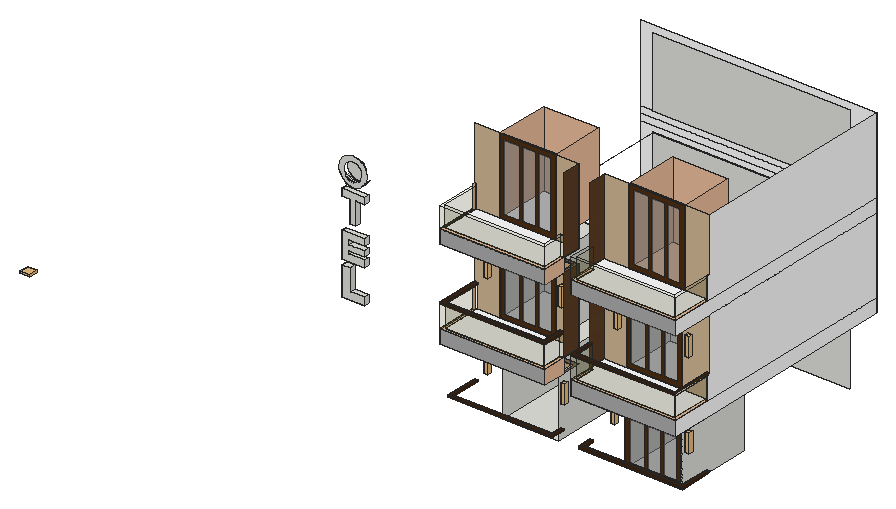
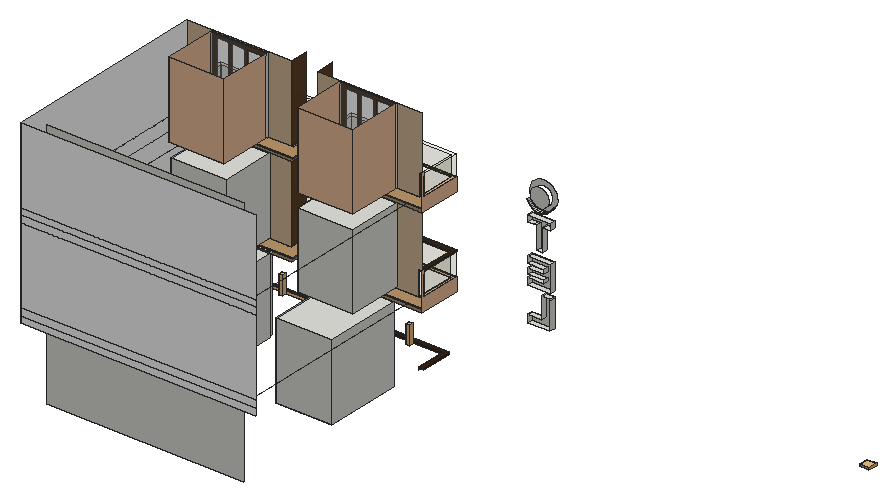
# SketchUp Ruby script. Lengths in inches.
U = 1.inch
M = Sketchup.active_model
def pt(a) = Geom::Point3d.new(a.map { |v| v * U })
def face(e, loops, mat)
  f = e.add_face(loops[0].map { |a| pt(a) })
  loops[1..].each { |l| e.add_face(l.map { |a| pt(a) }).erase! }
  f.material = f.back_material = mat if mat
  f
end
# faces: each face lists its corners as indices into pts; further lists are holes
def faces(e, pts, list, mat = nil) = list.each { |f| face(e, (f[0].is_a?(Array) ? f : [f]).map { |l| l.map { |i| pts[i] } }, mat) }
# xy, xz, yz: faces in a plane at the given z, y or x. An outline is a flat list of corners, or four numbers for a rectangle; further outlines are holes
def ring(l) = l.size == 4 ? [[l[0], l[1]], [l[2], l[1]], [l[2], l[3]], [l[0], l[3]]] : l.each_slice(2).to_a
def flat(e, list, mat, &to3) = list.each { |f| face(e, (f[0].is_a?(Array) ? f : [f]).map { |l| ring(l).map { |u, v| to3.(u, v) } }, mat) }
def xy(e, z, list, mat = nil) = flat(e, list, mat) { |x, y| [x, y, z] }
def xz(e, y, list, mat = nil) = flat(e, list, mat) { |x, z| [x, y, z] }
def yz(e, x, list, mat = nil) = flat(e, list, mat) { |y, z| [x, y, z] }
def lines(e, pts, list) = list.each { |a, b| e.add_line(pt(pts[a]), pt(pts[b])) }
# prism: a flat outline (further loops are holes) pulled along v
def prism(e, loops, v, mat = nil)
  f = face(e, loops, mat); d = Geom::Vector3d.new(v.map { |x| x * U })
  f.pushpull(f.normal.samedirection?(d) ? d.length : -d.length)
end
def box(e, o, s, mat = nil) = prism(e, [[o, [o[0] + s[0], o[1], o[2]], [o[0] + s[0], o[1] + s[1], o[2]], [o[0], o[1] + s[1], o[2]]]], [0, 0, s[2]], mat)
def at(x, y, z, deg = 0) = Geom::Transformation.translation(pt([x, y, z])) * Geom::Transformation.rotation(ORIGIN, Z_AXIS, deg.degrees)
def axes(o, x, y, z) = Geom::Transformation.new([*x, 0, *y, 0, *z, 0, *pt(o).to_a, 1])
def part(name) = M.definitions.add(name)
# library, detail: a bought-in or finely detailed component or shape, given as its bounding box
def library(name, o, s) = part(name).tap { |d| box(d.entities, o, s) }
def detail(e, o, s) = box(e.add_group.entities, o, s)
def put(e, d, t, mat = nil) = e.add_instance(d, t).tap { |i| i.material = mat if mat }
def group(e, t, mat = nil) = e.add_group.tap { |g| g.transformation = t; g.material = mat if mat }.entities
root = M.entities
M.materials.add("Generic").color = [68, 36, 11]
M.materials.add("Generic\#10").color = [214, 187, 153]
M.materials.add("Generic\#13").color = [239, 192, 158]
M.materials.add("Generic\#4").color = [186, 149, 106]
M.materials.add("Generic\#5").color = [175, 175, 175]
M.materials.add("Generic\#6").color = [117, 101, 81]
M.materials.add("[Color M00]").color = [255, 255, 255]
M.materials.add("[Translucent Glass Dark Green]").color = [86, 83, 28]
M.materials["[Translucent Glass Dark Green]"].alpha = 0.11
M.materials.add("[Translucent Glass Gray]1").color = [127, 127, 127]
M.materials["[Translucent Glass Gray]1"].alpha = 0.3
M.materials.add("[Wood Bamboo]").color = [81, 48, 19]
M.materials.add("[Wood Floor]").color = [91, 62, 36]
M.materials["[Wood Floor]"].alpha = 0.99
c1 = part("Group\#13")
xy(c1.entities,0,[[0,0,104.75,3]])
xy(c1.entities,142.8125,[[0,0,104.75,3]])
xz(c1.entities,0,[[8.08,8.08,37.11,134.73],[42.61,8.08,67.14,134.73],[72.39,8.08,96.67,134.73]],"[Translucent Glass Gray]1")
xz(c1.entities,0,[[[0,0,104.75,142.8125],[8.08,8.08,37.11,134.73],[42.61,8.08,67.14,134.73],[72.39,8.08,96.67,134.73]]],"[Wood Bamboo]")
xz(c1.entities,3,[[0,0,104.75,142.8125]],"[Translucent Glass Gray]1")
yz(c1.entities,0,[[0,0,3,142.8125]])
yz(c1.entities,104.75,[[0,0,3,142.8125]])
c2 = library("Tlon Light 450 Ceiling 152 006",[-8.86,-8.86,-3.78],[17.72,17.72,3.56])
c3 = library("Wall Lamp 298 005",[-4.37,-9,-20.45],[8.74,9.125,40.9])
xy(root,327.5625,[[458.2,140.75,562.95,286.875],[691.2,140.75,795.95,286.875]])
xy(root,372.75,[[404,78.3125,404,136.9375,409.82,136.9375,409.82,83.375,598,83.375,598,104.5,601.0625,104.5,601.0625,78.3125],[596.875,83.375,598,104.5]])
xy(root,372.75,[[650.9375,78.3125,650.9375,104.5,656.9375,104.5,656.9375,84.3125,842.4375,84.3125,842.4375,136.9375,848.4375,136.9375,848.4375,78.3125]],"Generic\#13")
xy(root,377.0625,[[404,78.3125,601.0625,78.3125,601.0625,104.5,596.875,104.5,596.875,83.375,409.82,83.375,409.82,140.75,404,140.75],[650.9375,78.3125,848.4375,78.3125,848.4375,136.9375,842.4375,136.9375,842.4375,84.3125,656.9375,84.3125,656.9375,104.5,650.9375,104.5],[842.4375,136.9375,848,140.75]],"Generic")
xy(root,470.375,[[458.2,140.75,562.95,286.875],[691.2,140.75,795.95,286.875]])
xy(root,470.375,[[[404,60.0625,601.0625,140.75],[409.34,65.4,595.73,131.6]],[[650.9375,60.0625,848,140.75],[655.73,64.86,843.21,132.14]]],"Generic\#6")
xy(root,471.6875,[[655.73,64.86,843.21,132.14],[409.34,65.4,595.73,131.6]],"Generic\#4")
xy(root,479.87,[[212.59,68.3125,254.57,78.3125]])
xy(root,494.05,[[228.04,68.3125,254.73,78.3125]])
xy(root,496.125,[[404,60.0625,404,136.9375,410,136.9375,410,66.0625,595.0625,66.0625,595.0625,104.5,601.0625,104.5,601.0625,60.0625],[650.9375,60.0625,650.9375,104.5,657.5625,104.5,657.5625,66.0625,842,66.0625,842,136.9375,848,136.9375,848,60.0625]],"Generic\#13")
xy(root,496.125,[[410,66.0625,595.0625,66.0625,595.0625,104.5,601.0625,104.5,601.0625,140.75,410,140.75],[657.5625,66.0625,842,66.0625,842,140.75,650.9375,140.75,650.9375,104.5,657.5625,104.5]],"[Color M00]")
xy(root,497.125,[[452.52,140.75,557.27,243.1875],[691.2,140.75,795.95,243.1875]])
xy(root,534.23,[[212.45,68.3125,227.88,78.3125]])
xy(root,538.125,[[404,60.0625,404,136.9375,410,136.9375,410,66.0625,595.0625,66.0625,595.0625,104.5,601.0625,104.5,601.0625,60.0625],[650.9375,60.0625,650.9375,104.5,657.5625,104.5,657.5625,66.0625,842,66.0625,842,136.9375,848,136.9375,848,60.0625]])
xy(root,541.4375,[[404,60.0625,601.0625,60.0625,601.0625,104.5,595.0625,104.5,595.0625,66.0625,410,66.0625,410,140.75,404,140.75],[650.9375,60.0625,848,60.0625,848,140.75,842,140.75,842,66.0625,657.5625,66.0625,657.5625,104.5,650.9375,104.5]],"Generic")
xy(root,543.68,[[212.13,68.3125,254.57,78.3125]])
xy(root,556.18,[[224.88,68.3125,254.57,78.3125]])
xy(root,561.8,[[224.88,68.3125,254.57,78.3125]])
xy(root,572.3,[[224.88,68.3125,254.57,78.3125]])
xy(root,579.92,[[224.88,68.3125,254.57,78.3125]])
xy(root,592.36,[[212.13,68.3125,254.57,78.3125]])
xy(root,608.06,[[226.26,68.3125,238.26,78.3125]])
xy(root,640.125,[[452.52,140.75,557.27,243.1875],[691.2,140.75,795.95,243.1875]])
xy(root,640.125,[[[404,60.0625,601.0625,140.75],[408.75,64.8125,596.3125,132.1875]],[[650.9375,60.0625,848,140.75],[655.28,64.4,843.66,132.6]]],"Generic\#6")
xy(root,641.4375,[[655.28,64.4,843.66,132.6],[408.75,64.8125,596.3125,132.1875]],"Generic\#4")
xy(root,650.42,[[210.88,68.3125,226.26,78.3125],[238.26,68.3125,242.57,78.3125],[242.57,68.3125,254.57,78.3125]])
xy(root,662.42,[[210.88,68.3125,254.57,78.3125]])
xy(root,665.875,[[404,60.0625,404,136.9375,408.8125,136.9375,408.8125,66.0625,596,66.0625,596,104.5,601.0625,104.5,601.0625,60.0625],[650.9375,60.0625,650.9375,104.5,657.6875,104.5,657.6875,66.0625,842,66.0625,842,136.9375,848,136.9375,848,60.0625],[696.14,140.75,800.89,243.1875]],"Generic\#13")
xy(root,665.875,[[408.8125,66.0625,596,66.0625,596,104.5,601.0625,104.5,601.0625,140.75,557.27,140.75,557.27,243.1875,452.52,243.1875,452.52,140.75,408.8125,140.75],[657.6875,66.0625,842,66.0625,842,140.75,650.9375,140.75,650.9375,104.5,657.6875,104.5]],"[Color M00]")
xz(root,60.0625,[[404,538.125,601.0625,541.4375],[650.9375,538.125,848,541.4375]],"Generic")
xz(root,60.0625,[[404,470.375,601.0625,496.125],[650.9375,470.375,848,496.125],[404,640.125,601.0625,665.875],[650.9375,640.125,848,665.875]],"Generic\#5")
xz(root,60.0625,[[404,496.125,601.0625,538.125],[650.9375,496.125,848,538.125],[404,665.875,601.0625,704.1875],[650.9375,665.875,848,704.1875]],"[Translucent Glass Dark Green]")
xz(root,64.4,[[655.28,640.125,843.66,641.4375]])
xz(root,64.8125,[[408.75,640.125,596.3125,641.4375]])
xz(root,64.86,[[655.73,470.375,843.21,471.6875]])
xz(root,65.4,[[409.34,470.375,595.73,471.6875]])
xz(root,66.0625,[[410,538.125,595.0625,541.4375],[657.5625,538.125,842,541.4375]],"Generic")
xz(root,66.0625,[[410,496.125,595.0625,538.125],[657.5625,496.125,842,538.125],[408.8125,665.875,596,704.1875],[657.6875,665.875,842,704.1875]],"[Translucent Glass Dark Green]")
xz(root,68.3125,[[212.59,479.87,254.57,479.87,254.73,494.05,228.04,494.05,227.88,534.23,212.45,534.23,212.59,531.7],[212.13,543.68,254.57,543.68,254.57,556.18,224.88,556.18,224.88,561.8,254.57,561.8,254.57,572.3,224.88,572.3,224.88,579.92,254.57,579.92,254.57,592.36,212.13,592.36],[226.26,608.06,238.26,608.06,238.26,650.42,254.57,650.42,254.57,662.42,210.88,662.42,210.88,650.42,226.26,650.42],[[233.53,671.96,236.44,672.22,239.27,672.93,242.09,673.69,244.76,674.89,247.27,676.38,249.6,678.15,251.72,680.16,253.6,682.4,255.21,684.83,256.55,687.44,257.58,690.17,258.3,693,258.7,695.9,258.78,698.82,258.52,701.73,257.95,704.59,257.05,707.375,255.85,710.04,254.36,712.55,252.59,714.88,250.58,717,248.34,718.88,245.91,720.5,243.3,721.83,240.57,722.87,237.74,723.59,234.84,723.99,231.92,724.0625,229.01,723.81,226.15,723.23,223.36,722.33,220.7,721.13,218.1875,719.64,215.86,717.88,213.74,715.86,211.86,713.625,210.24,711.19,208.91,708.59,207.875,705.86,207.15,703.02,206.75,700.13,206.68,697.21,206.93,694.3,207.51,691.43,208.4,688.65,209.61,685.98,211.1,683.47,212.86,681.14,214.875,679.02,217.11,677.14,219.55,675.53,222.15,674.19,224.88,673.16,227.72,672.4375,230.61,672.04],[233.26,680.77,231.33,680.82,229.41,681.08,227.53,681.56,225.73,682.24,224,683.13,222.39,684.2,220.91,685.44,219.58,686.84,218.41,688.39,217.42,690.05,216.625,691.8125,216.03,693.66,215.65,695.55,215.48,697.48,215.53,699.41,215.8,701.33,216.27,703.21,216.96,705.01,217.84,706.74,218.91,708.35,220.16,709.83,221.56,711.16,223.1,712.33,224.76,713.32,226.53,714.11,228.37,714.71,230.27,715.09,232.19,715.26,234.13,715.21,236.05,714.94,237.92,714.47,239.73,713.78,241.45,712.9,243.0625,711.83,244.54,710.58,245.88,709.18,247.05,707.64,248.03,705.98,248.83,704.21,249.42,702.37,249.8,700.47,249.97,698.55,249.92,696.61,249.66,694.69,249.18,692.82,248.5,691.01,247.61,689.29,246.54,687.68,245.3,686.2,243.9,684.86,242.35,683.69,240.69,682.71,239.12,682,237.05,681.44,234.97,680.92]]])
xz(root,78.3125,[[233.26,680.77,234.97,680.92,237.05,681.44,239.12,682,240.69,682.71,242.35,683.69,243.9,684.86,245.3,686.2,246.54,687.68,247.61,689.29,248.5,691.01,249.18,692.82,249.66,694.69,249.92,696.61,249.97,698.55,249.8,700.47,249.42,702.37,248.83,704.21,248.03,705.98,247.05,707.64,245.88,709.18,244.54,710.58,243.0625,711.83,241.45,712.9,239.73,713.78,237.92,714.47,236.05,714.94,234.13,715.21,232.19,715.26,230.27,715.09,228.37,714.71,226.53,714.11,224.76,713.32,223.1,712.33,221.56,711.16,220.16,709.83,218.91,708.35,217.84,706.74,216.96,705.01,216.27,703.21,215.8,701.33,215.53,699.41,215.48,697.48,215.65,695.55,216.03,693.66,216.625,691.8125,217.42,690.05,218.41,688.39,219.58,686.84,220.91,685.44,222.39,684.2,224,683.13,225.73,682.24,227.53,681.56,229.41,681.08,231.33,680.82]])
xz(root,78.3125,[[404,372.75,601.0625,377.0625],[650.9375,372.75,848.4375,377.0625]],"Generic")
xz(root,83.375,[[409.82,372.75,596.875,377.0625]],"Generic")
xz(root,84.3125,[[656.9375,372.75,842.4375,377.0625]],"Generic\#13")
xz(root,104.5,[[596.875,372.75,601.0625,377.0625],[595.0625,538.125,601.0625,541.4375],[650.9375,538.125,657.5625,541.4375]])
xz(root,104.5,[[650.9375,372.75,656.9375,377.0625]],"Generic\#13")
xz(root,104.5,[[595.0625,496.125,601.0625,538.125],[650.9375,496.125,657.5625,538.125],[596,665.875,601.0625,704.1875],[650.9375,665.875,657.6875,704.1875]],"[Translucent Glass Dark Green]")
xz(root,131.6,[[409.34,470.375,440,471.6875],[440,470.375,595.73,471.6875]],"Generic\#6")
xz(root,132.14,[[655.73,470.375,812,471.6875],[812,470.375,843.21,471.6875]],"Generic\#6")
xz(root,132.1875,[[408.75,640.125,440,641.4375]])
xz(root,132.1875,[[440,640.125,596.3125,641.4375]],"Generic\#6")
xz(root,132.6,[[655.28,640.125,843.66,641.4375]],"Generic\#6")
xz(root,136.9375,[[842.4375,372.75,848,377.0625],[848,372.75,848.4375,377.0625]],"Generic\#13")
xz(root,140.75,[[458.2,470.375,562.95,470.5625],[691.2,470.375,795.95,470.5625],[452.52,640.125,557.27,640.1875],[691.2,640.125,795.95,640.1875]])
xz(root,140.75,[[410,496.125,601.0625,496.125,601.0625,640.125,557.27,640.125,557.27,497.125,452.52,497.125,452.52,640.125,404,640.125,404,541.4375,410,541.4375],[650.9375,496.125,842,496.125,842,541.4375,848,541.4375,848,640.125,795.95,640.125,795.95,497.125,691.2,497.125,691.2,640.125,650.9375,640.125],[408.8125,665.875,452.52,665.875,452.52,808.9375,557.27,808.9375,557.27,665.875,601.0625,665.875,601.0625,809.875,404,809.875,404,708.0625,408.8125,708.0625],[650.9375,665.875,696.14,665.875,696.14,808.9375,800.89,808.9375,800.89,665.875,842,665.875,842,708.0625,848,708.0625,848,809.875,650.9375,809.875]],"Generic\#10")
xz(root,140.75,[[696.14,664.9375,800.89,665.875]],"Generic\#13")
xz(root,243.1875,[[452.52,497.125,557.27,640.125],[691.2,497.125,795.95,640.125]])
xz(root,243.1875,[[452.52,665.875,557.27,808.9375],[696.14,665.875,800.89,808.9375]],"Generic\#13")
xz(root,286.875,[[458.2,327.5625,562.95,470.375],[691.2,327.5625,795.95,470.375]])
xz(root,515.9375,[[440,338,812,470.375],[440,507.75,812,640.125],[440,677.5,812,809.875]])
xz(root,534.3125,[[404,470.375,848,483.5],[404,483.5,848,496.125],[404,496.125,848,640.125],[404,640.125,848,653.25],[404,653.25,848,665.875],
  [404,665.875,848,809.875]],"[Color M00]")
yz(root,210.88,[[68.3125,650.42,78.3125,662.42]])
yz(root,212.13,[[68.3125,543.68,78.3125,592.36]])
yz(root,212.59,[[68.3125,479.87,78.3125,531.7]])
yz(root,224.88,[[68.3125,556.18,78.3125,561.8],[68.3125,572.3,78.3125,579.92]])
yz(root,226.26,[[68.3125,608.06,78.3125,650.42]])
yz(root,238.26,[[68.3125,608.06,78.3125,650.42]])
yz(root,254.57,[[68.3125,543.68,78.3125,556.18],[68.3125,561.8,78.3125,572.3],[68.3125,579.92,78.3125,592.36],[68.3125,650.42,78.3125,662.42]])
yz(root,404,[[78.3125,372.75,136.9375,377.0625],[60.0625,538.125,136.9375,541.4375]],"Generic")
yz(root,404,[[60.0625,470.375,60.0625,496.125,136.9375,496.125,136.9375,541.4375,140.75,541.4375,140.75,470.375],[60.0625,640.125,60.0625,665.875,136.9375,665.875,136.9375,708.0625,140.75,708.0625,140.75,640.125]],"Generic\#13")
yz(root,404,[[60.0625,496.125,136.9375,538.125],[60.0625,665.875,136.9375,704.1875]],"[Translucent Glass Dark Green]")
yz(root,408.75,[[64.8125,640.125,132.1875,641.4375]],"Generic\#6")
yz(root,408.8125,[[66.0625,665.875,140.75,704.1875]],"[Translucent Glass Dark Green]")
yz(root,409.34,[[65.4,470.375,131.6,471.6875]])
yz(root,409.82,[[83.375,372.75,140.75,377.0625]],"Generic")
yz(root,410,[[66.0625,538.125,140.75,541.4375]],"Generic")
yz(root,410,[[66.0625,496.125,140.75,538.125]],"[Translucent Glass Dark Green]")
yz(root,452.52,[[140.75,497.125,243.1875,640.125]])
yz(root,452.52,[[140.75,665.875,243.1875,808.9375]],"Generic\#13")
yz(root,458.2,[[140.75,327.5625,286.875,470.375]])
yz(root,557.27,[[140.75,497.125,243.1875,640.125]])
yz(root,557.27,[[140.75,665.875,243.1875,808.9375]],"Generic\#13")
yz(root,562.95,[[140.75,327.5625,286.875,470.375]])
yz(root,595.0625,[[66.0625,538.125,104.5,541.4375]],"Generic")
yz(root,595.0625,[[66.0625,496.125,104.5,538.125]],"[Translucent Glass Dark Green]")
yz(root,595.73,[[65.4,470.375,104.5,471.6875],[104.5,470.375,131.6,471.6875]])
yz(root,596,[[66.0625,665.875,104.5,704.1875]],"[Translucent Glass Dark Green]")
yz(root,596.3125,[[64.8125,640.125,104.5,641.4375],[104.5,640.125,132.1875,641.4375]],"Generic\#6")
yz(root,596.875,[[83.375,372.75,104.5,377.0625]],"Generic")
yz(root,601.0625,[[78.3125,372.75,104.5,377.0625],[60.0625,538.125,104.5,541.4375]],"Generic")
yz(root,601.0625,[[60.0625,470.375,104.5,496.125],[60.0625,640.125,104.5,665.875]],"Generic\#13")
yz(root,601.0625,[[60.0625,496.125,104.5,538.125],[60.0625,665.875,104.5,704.1875]],"[Translucent Glass Dark Green]")
yz(root,601.0625,[[104.5,496.125,140.75,640.125],[104.5,665.875,140.75,809.875]],"[Wood Floor]")
yz(root,650.9375,[[78.3125,372.75,104.5,377.0625],[60.0625,538.125,104.5,541.4375]],"Generic")
yz(root,650.9375,[[60.0625,470.375,104.5,496.125],[60.0625,640.125,104.5,665.875]],"Generic\#13")
yz(root,650.9375,[[60.0625,496.125,104.5,538.125],[60.0625,665.875,104.5,704.1875]],"[Translucent Glass Dark Green]")
yz(root,650.9375,[[104.5,496.125,140.75,640.125],[104.5,665.875,140.75,809.875]],"[Wood Floor]")
yz(root,655.28,[[64.4,640.125,132.6,641.4375]],"Generic\#6")
yz(root,655.73,[[64.86,470.375,104.5,471.6875],[104.5,470.375,132.14,471.6875]],"Generic\#6")
yz(root,656.9375,[[84.3125,372.75,104.5,377.0625]],"Generic")
yz(root,657.5625,[[66.0625,538.125,104.5,541.4375]],"Generic")
yz(root,657.5625,[[66.0625,496.125,104.5,538.125]],"[Translucent Glass Dark Green]")
yz(root,657.6875,[[66.0625,665.875,104.5,704.1875]],"[Translucent Glass Dark Green]")
yz(root,691.2,[[140.75,327.5625,286.875,470.375],[140.75,497.125,243.1875,640.125]])
yz(root,696.14,[[140.75,665.875,243.1875,808.9375]],"Generic\#13")
yz(root,795.95,[[140.75,327.5625,286.875,470.375],[140.75,497.125,243.1875,640.125]])
yz(root,800.89,[[140.75,665.875,243.1875,808.9375]],"Generic\#13")
yz(root,842,[[66.0625,538.125,140.75,541.4375]],"Generic")
yz(root,842,[[66.0625,496.125,140.75,538.125],[66.0625,665.875,140.75,704.1875]],"[Translucent Glass Dark Green]")
yz(root,842.4375,[[84.3125,372.75,136.9375,377.0625]],"Generic")
yz(root,842.4375,[[136.9375,372.75,140.75,377.0625]],"Generic\#13")
yz(root,843.21,[[64.86,470.375,132.14,471.6875]],"Generic\#6")
yz(root,843.66,[[64.4,640.125,132.6,641.4375]],"Generic\#6")
yz(root,848,[[60.0625,538.125,136.9375,541.4375]])
yz(root,848,[[60.0625,470.375,534.3125,496.125],[136.9375,496.125,534.3125,496.125,534.3125,640.125,140.75,640.125,140.75,541.4375,136.9375,541.4375],[60.0625,640.125,534.3125,665.875],[136.9375,665.875,534.3125,665.875,534.3125,809.875,140.75,809.875,140.75,708.0625,136.9375,708.0625]],"[Color M00]")
yz(root,848,[[60.0625,496.125,136.9375,538.125],[60.0625,665.875,136.9375,704.1875]],"[Translucent Glass Dark Green]")
yz(root,848.4375,[[78.3125,372.75,136.9375,377.0625]],"Generic")
p = [[254.57,78.3125,479.87],[254.73,78.3125,494.05],[254.73,68.3125,494.05],[254.57,68.3125,479.87],[228.04,78.3125,494.05],[227.88,78.3125,534.23],
  [227.88,68.3125,534.23],[228.04,68.3125,494.05],[212.45,78.3125,534.23],[212.59,78.3125,531.7],[212.59,68.3125,531.7],[212.45,68.3125,534.23],
  [227.72,78.3125,672.4375],[230.61,78.3125,672.04],[230.61,68.3125,672.04],[227.72,68.3125,672.4375],[233.53,78.3125,671.96],[233.53,68.3125,671.96],
  [236.44,78.3125,672.22],[236.44,68.3125,672.22],[239.27,78.3125,672.93],[239.27,68.3125,672.93],[224.88,78.3125,673.16],[224.88,68.3125,673.16],
  [242.09,78.3125,673.69],[242.09,68.3125,673.69],[222.15,78.3125,674.19],[222.15,68.3125,674.19],[244.76,78.3125,674.89],[244.76,68.3125,674.89],
  [219.55,78.3125,675.53],[219.55,68.3125,675.53],[247.27,78.3125,676.38],[247.27,68.3125,676.38],[217.11,78.3125,677.14],[217.11,68.3125,677.14],
  [249.6,78.3125,678.15],[249.6,68.3125,678.15],[214.875,78.3125,679.02],[214.875,68.3125,679.02],[251.72,78.3125,680.16],[251.72,68.3125,680.16],
  [212.86,78.3125,681.14],[212.86,68.3125,681.14],[253.6,78.3125,682.4],[253.6,68.3125,682.4],[231.33,78.3125,680.82],[229.41,78.3125,681.08],
  [229.41,68.3125,681.08],[231.33,68.3125,680.82],[233.26,78.3125,680.77],[233.26,68.3125,680.77],[234.97,78.3125,680.92],[234.97,68.3125,680.92],
  [237.05,78.3125,681.44],[237.05,68.3125,681.44],[211.1,78.3125,683.47],[211.1,68.3125,683.47],[227.53,78.3125,681.56],[227.53,68.3125,681.56],
  [239.12,78.3125,682],[239.12,68.3125,682],[225.73,78.3125,682.24],[225.73,68.3125,682.24],[240.69,78.3125,682.71],[240.69,68.3125,682.71],
  [224,78.3125,683.13],[224,68.3125,683.13],[255.21,78.3125,684.83],[255.21,68.3125,684.83],[242.35,78.3125,683.69],[242.35,68.3125,683.69],
  [222.39,78.3125,684.2],[222.39,68.3125,684.2],[209.61,78.3125,685.98],[209.61,68.3125,685.98],[243.9,78.3125,684.86],[243.9,68.3125,684.86],
  [220.91,78.3125,685.44],[220.91,68.3125,685.44],[256.55,78.3125,687.44],[256.55,68.3125,687.44],[245.3,78.3125,686.2],[245.3,68.3125,686.2],
  [219.58,78.3125,686.84],[219.58,68.3125,686.84],[208.4,78.3125,688.65],[208.4,68.3125,688.65],[246.54,78.3125,687.68],[246.54,68.3125,687.68],
  [440,515.9375,472.9375],[812,515.9375,472.9375],[440,515.9375,642.6875],[812,515.9375,642.6875],[440,136.9375,640.125],[440,140.75,640.125],
  [812,136.9375,640.125],[812,140.75,640.125],[440,136.9375,470.375],[440,140.75,470.375],[812,136.9375,470.375],[812,140.75,470.375],
  [440,515.9375,640.125],[812,515.9375,640.125],[440,515.9375,470.375],[812,515.9375,470.375]]
faces(root,p,[[0,1,2,3],[4,5,6,7],[8,9,10,11],[12,13,14,15],[13,16,17,14],[16,18,19,17],[18,20,21,19],[22,12,15,23],
  [20,24,25,21],[26,22,23,27],[24,28,29,25],[30,26,27,31],[28,32,33,29],[34,30,31,35],[32,36,37,33],[38,34,35,39],
  [36,40,41,37],[42,38,39,43],[40,44,45,41],[46,47,48,49],[50,46,49,51],[52,50,51,53],[54,52,53,55],[56,42,43,57],
  [47,58,59,48],[60,54,55,61],[58,62,63,59],[64,60,61,65],[62,66,67,63],[44,68,69,45],[70,64,65,71],[66,72,73,67],
  [74,56,57,75],[76,70,71,77],[72,78,79,73],[68,80,81,69],[82,76,77,83],[78,84,85,79],[86,74,75,87],[88,82,83,89]])
lines(root,p,[[90,91],[92,93],[94,95],[96,97],[98,99],[100,101],[95,102],[97,103],[99,104],[101,105]])
put(root,c1,at(691.2,137.75,331.11))
put(root,c2,at(-299.52,-31.2,387.73))
put(root,c3,axes([436.94,134.14,419.74],[0.8568,0,0],[0,0.8568,0],[0,0,0.8568]))
put(root,c3,axes([582.01,134.14,419.74],[0.8568,0,0],[0,0.8568,0],[0,0,0.8568]))
put(root,c3,axes([676.76,134.14,419.74],[0.8568,0,0],[0,0.8568,0],[0,0,0.8568]))
put(root,c3,axes([817.19,134.14,419.74],[0.8568,0,0],[0,0.8568,0],[0,0,0.8568]))
put(root,c2,at(808.47,97.91,472.91))
put(root,c2,at(693.97,97.91,472.91))
put(root,c2,at(571.28,97.91,472.91))
put(root,c2,at(441.78,97.91,472.91))
put(root,c1,at(691.2,140.75,497.125))
put(root,c1,at(453.08,140.75,497.125))
put(root,c3,axes([816.88,134.14,582.68],[0.8568,0,0],[0,0.8568,0],[0,0,0.8568]))
put(root,c3,axes([682.94,134.14,582.68],[0.8568,0,0],[0,0.8568,0],[0,0,0.8568]))
put(root,c3,axes([577.57,134.14,582.68],[0.8568,0,0],[0,0.8568,0],[0,0,0.8568]))
put(root,c3,axes([436.94,134.14,582.68],[0.8568,0,0],[0,0.8568,0],[0,0,0.8568]))
put(root,c2,at(569.64,89.28,642.48))
put(root,c2,at(445.95,95.53,642.48))
put(root,c2,at(684.64,95.84,642.48))
put(root,c2,at(813.89,95.84,642.48))
put(root,c1,at(696.14,140.75,665.875))
put(root,c1,at(452.52,140.75,665.875))
